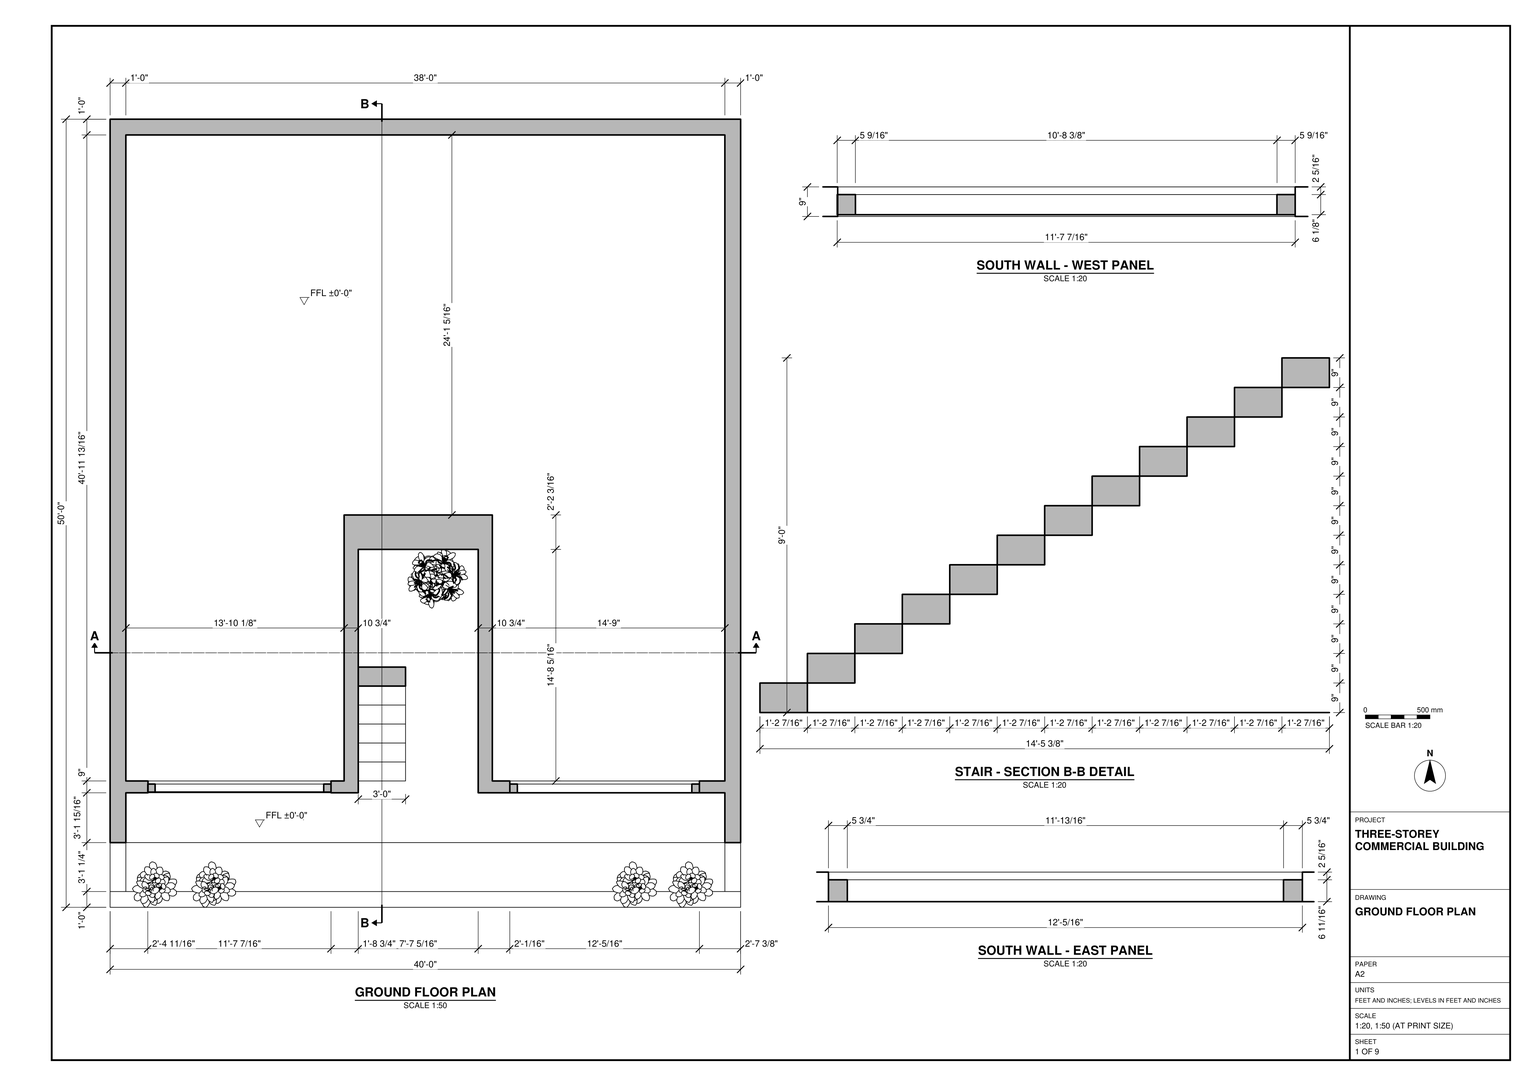
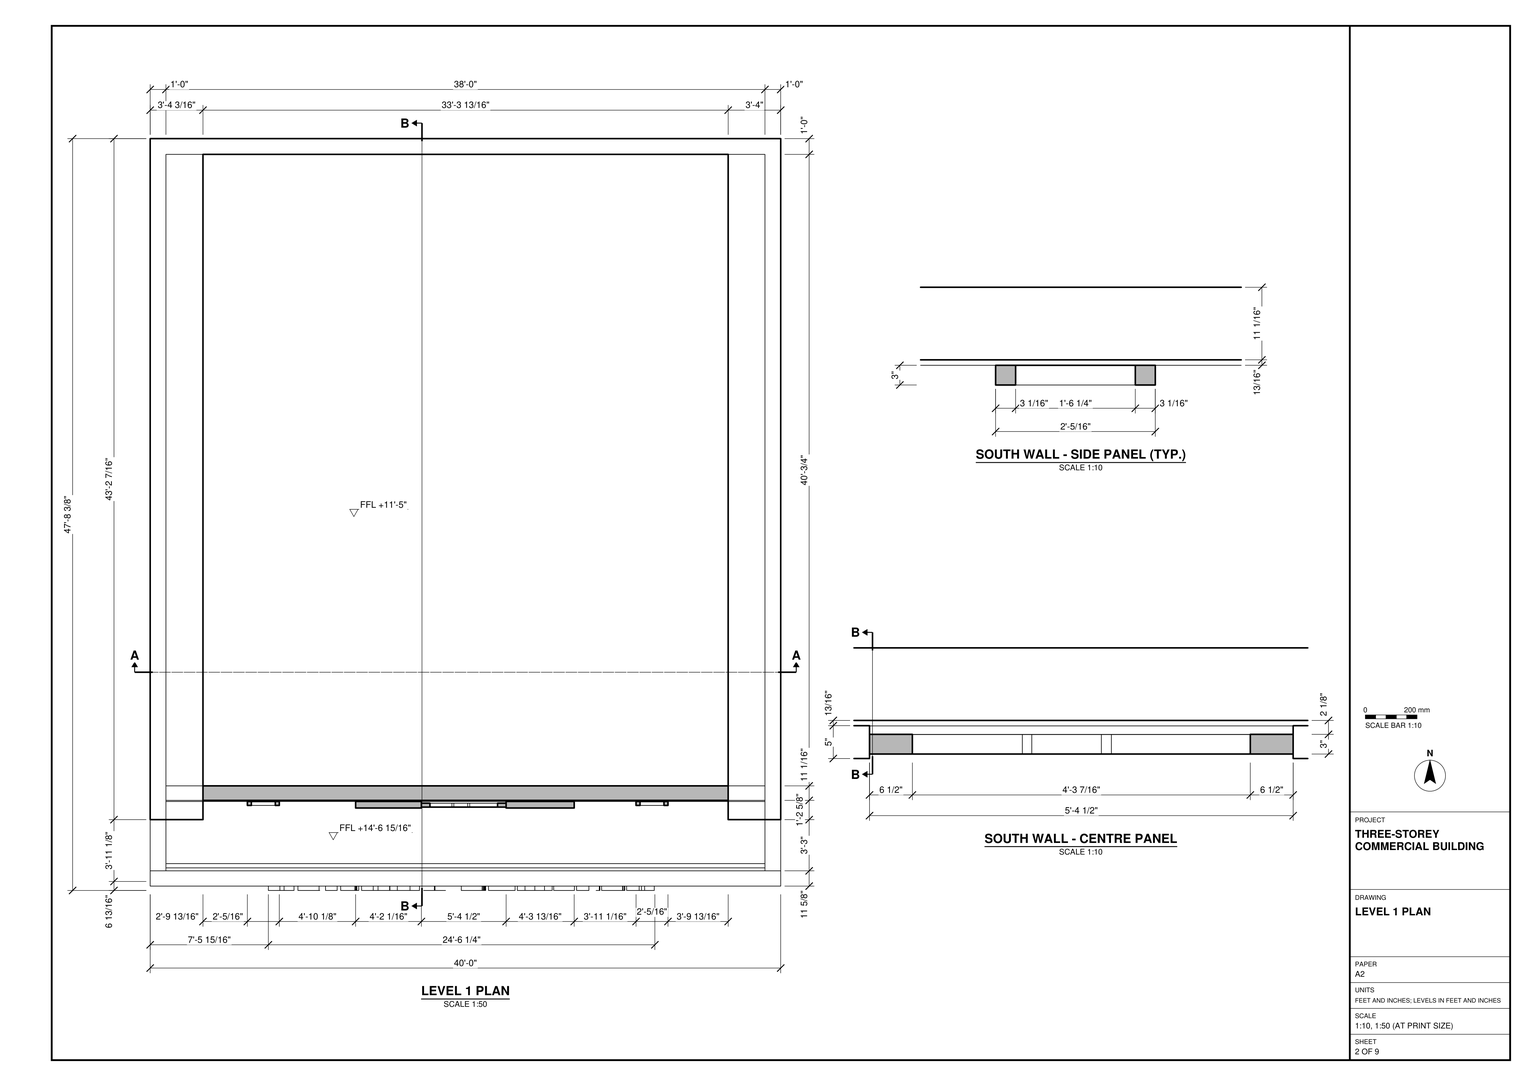
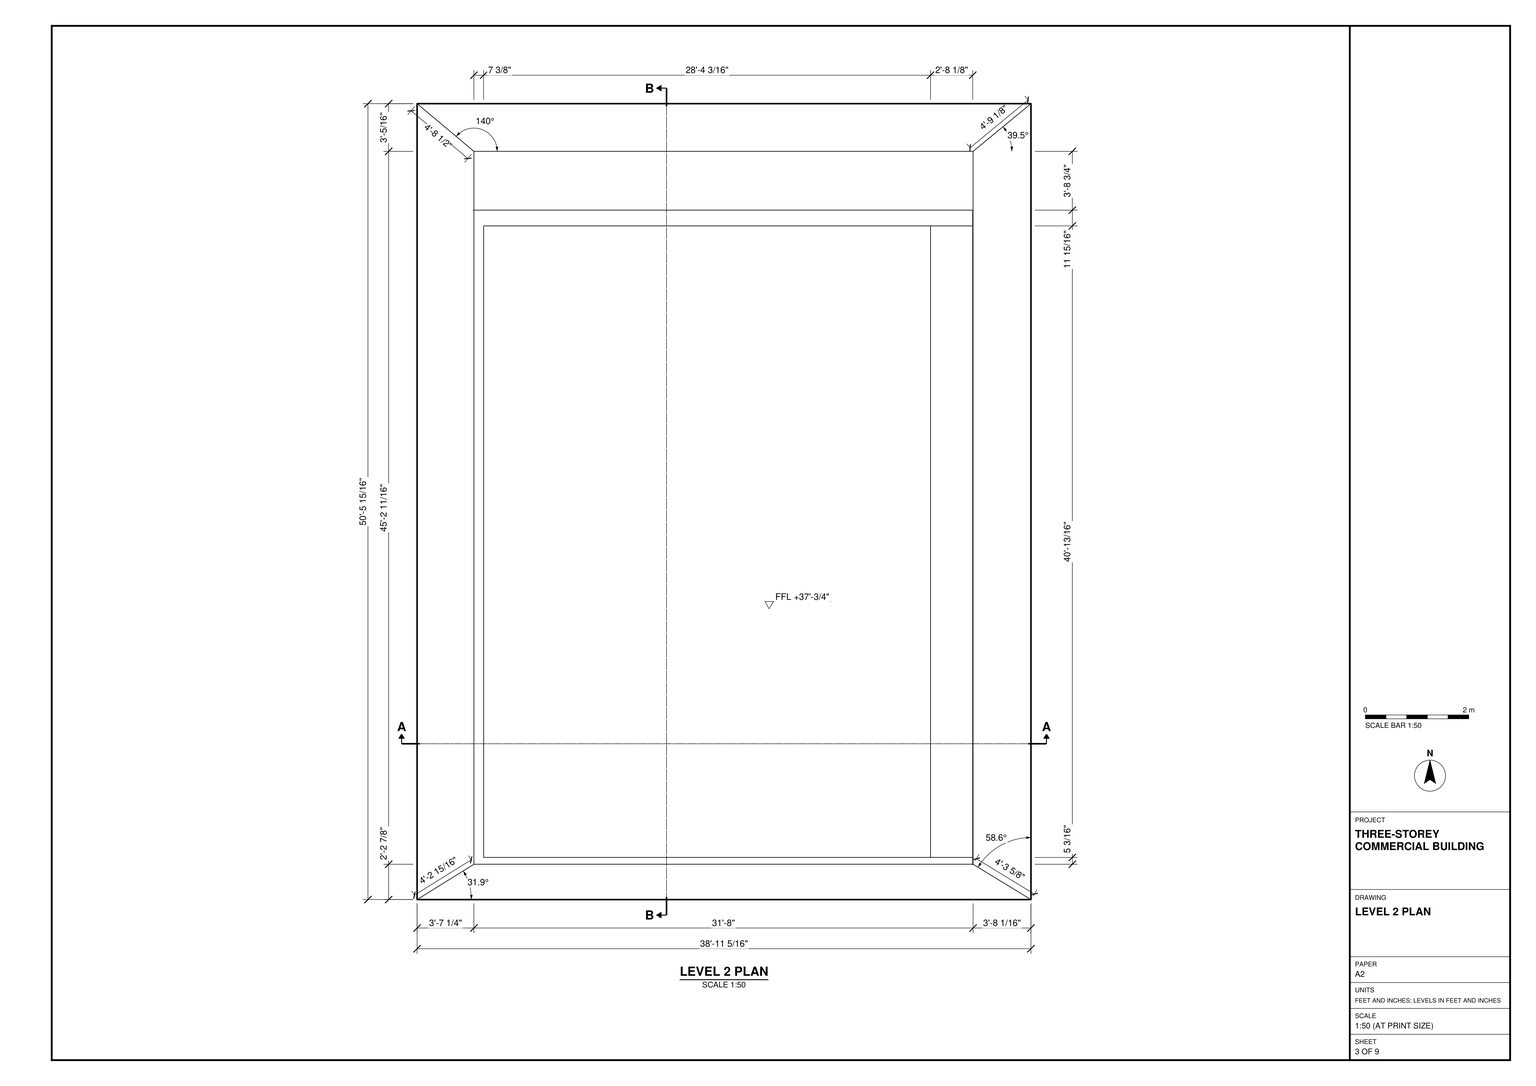
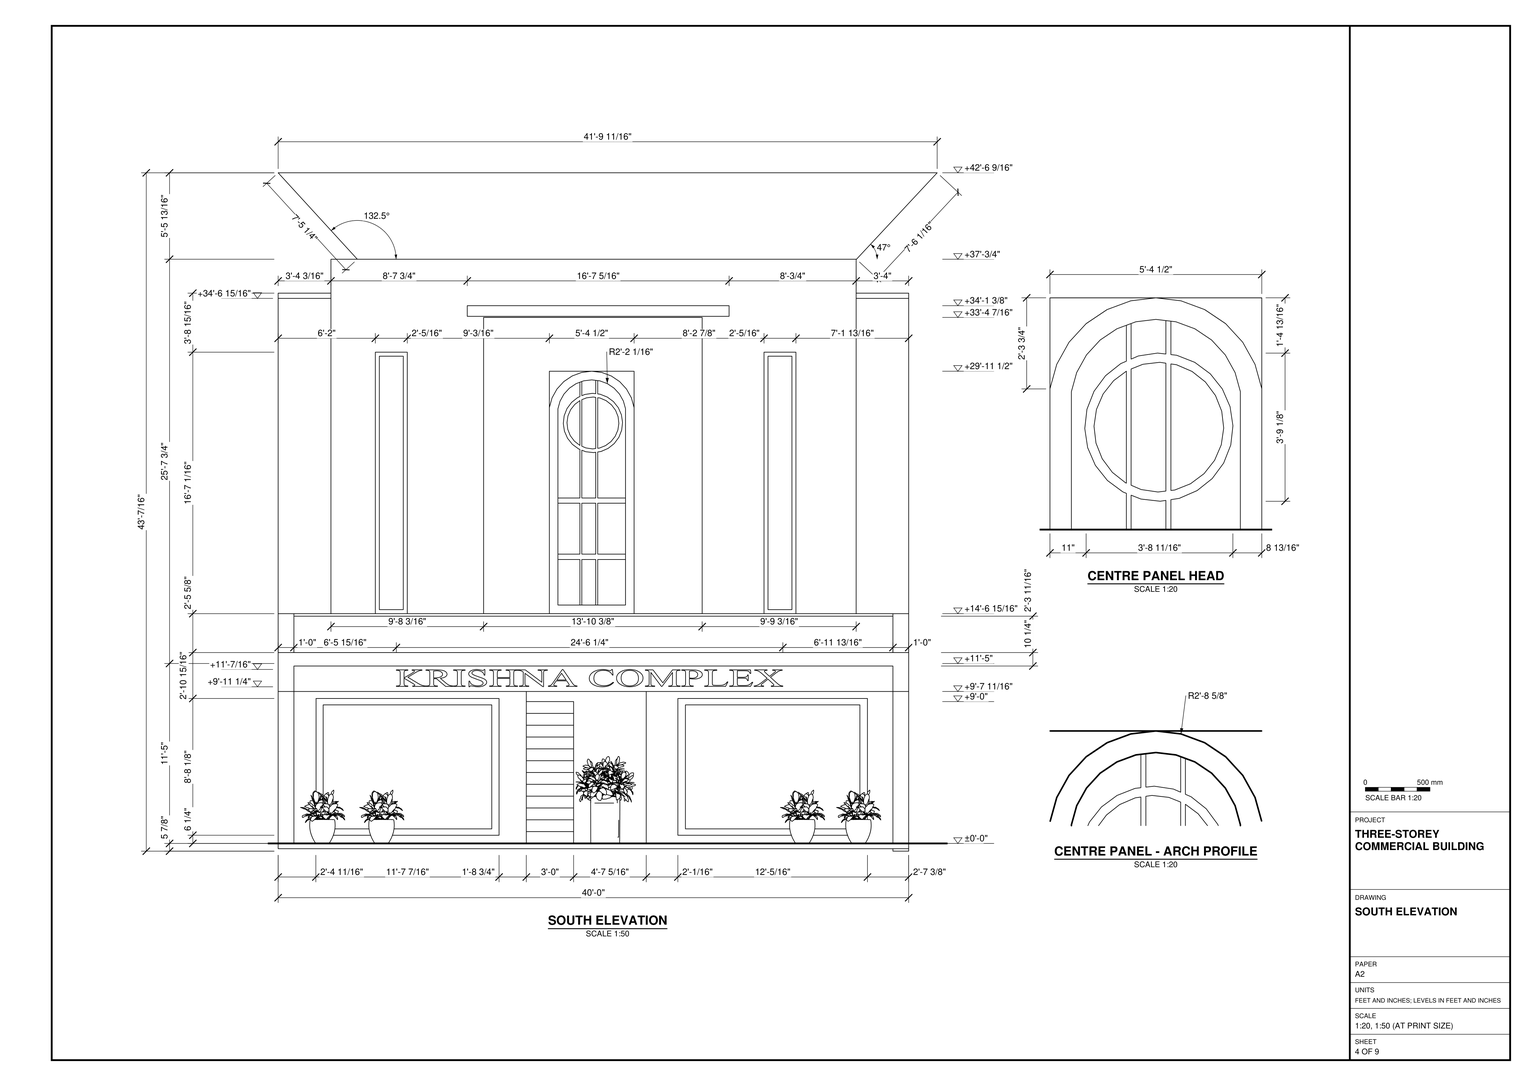
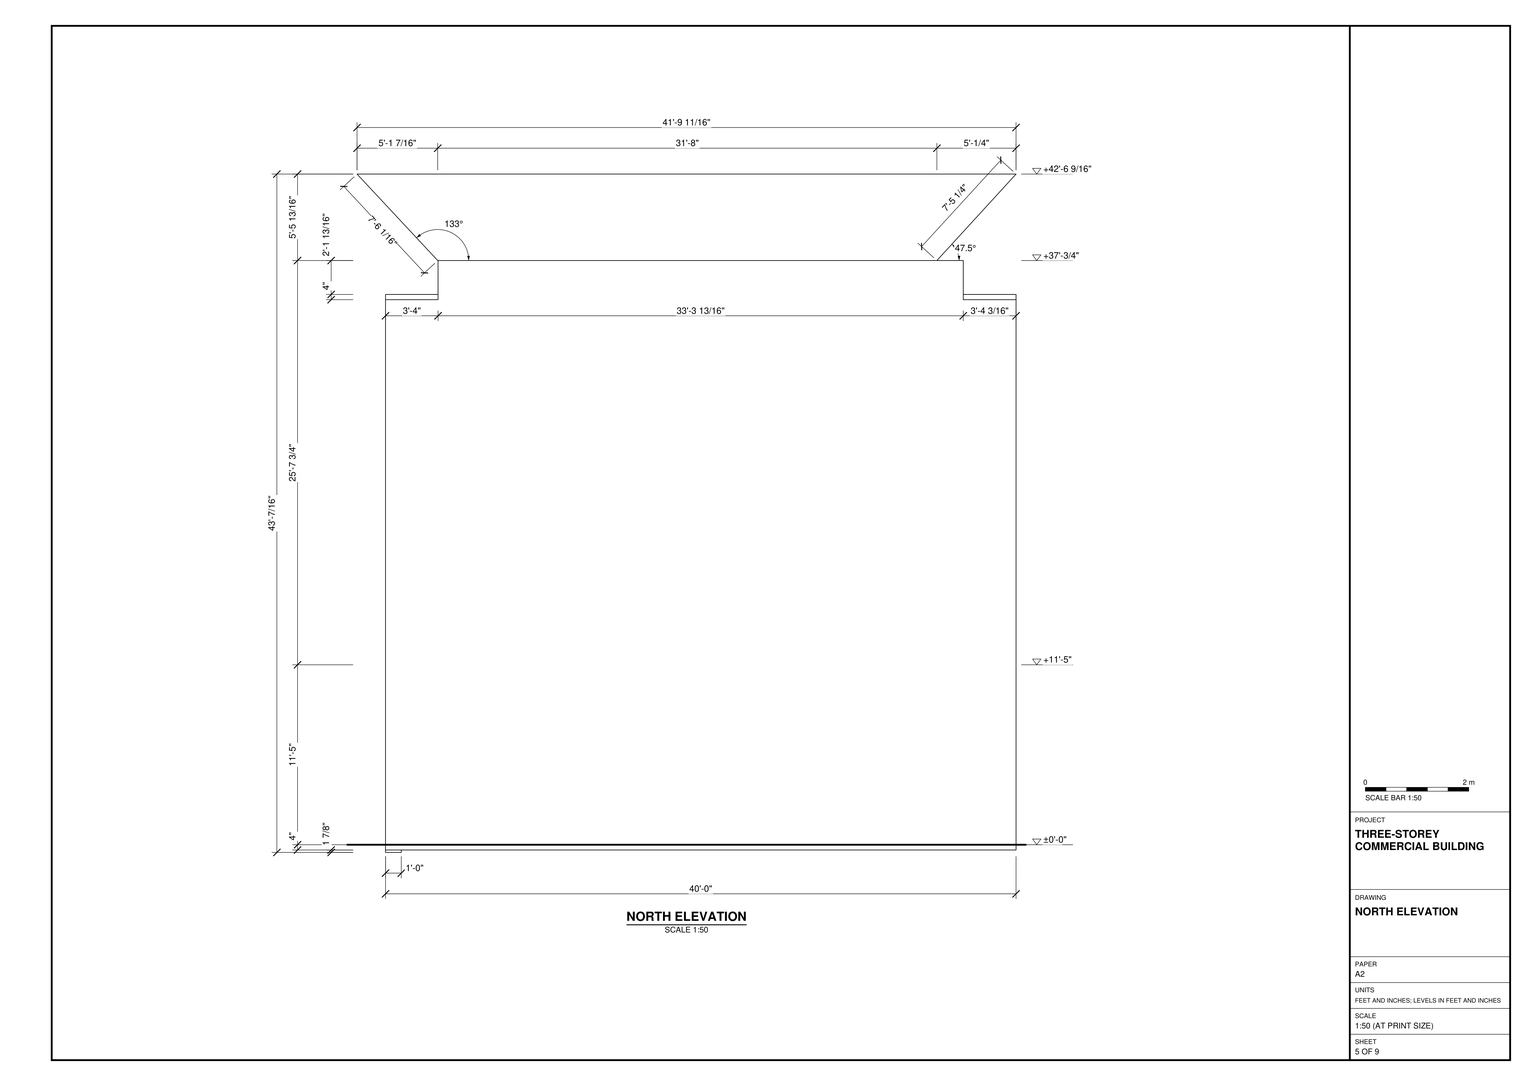
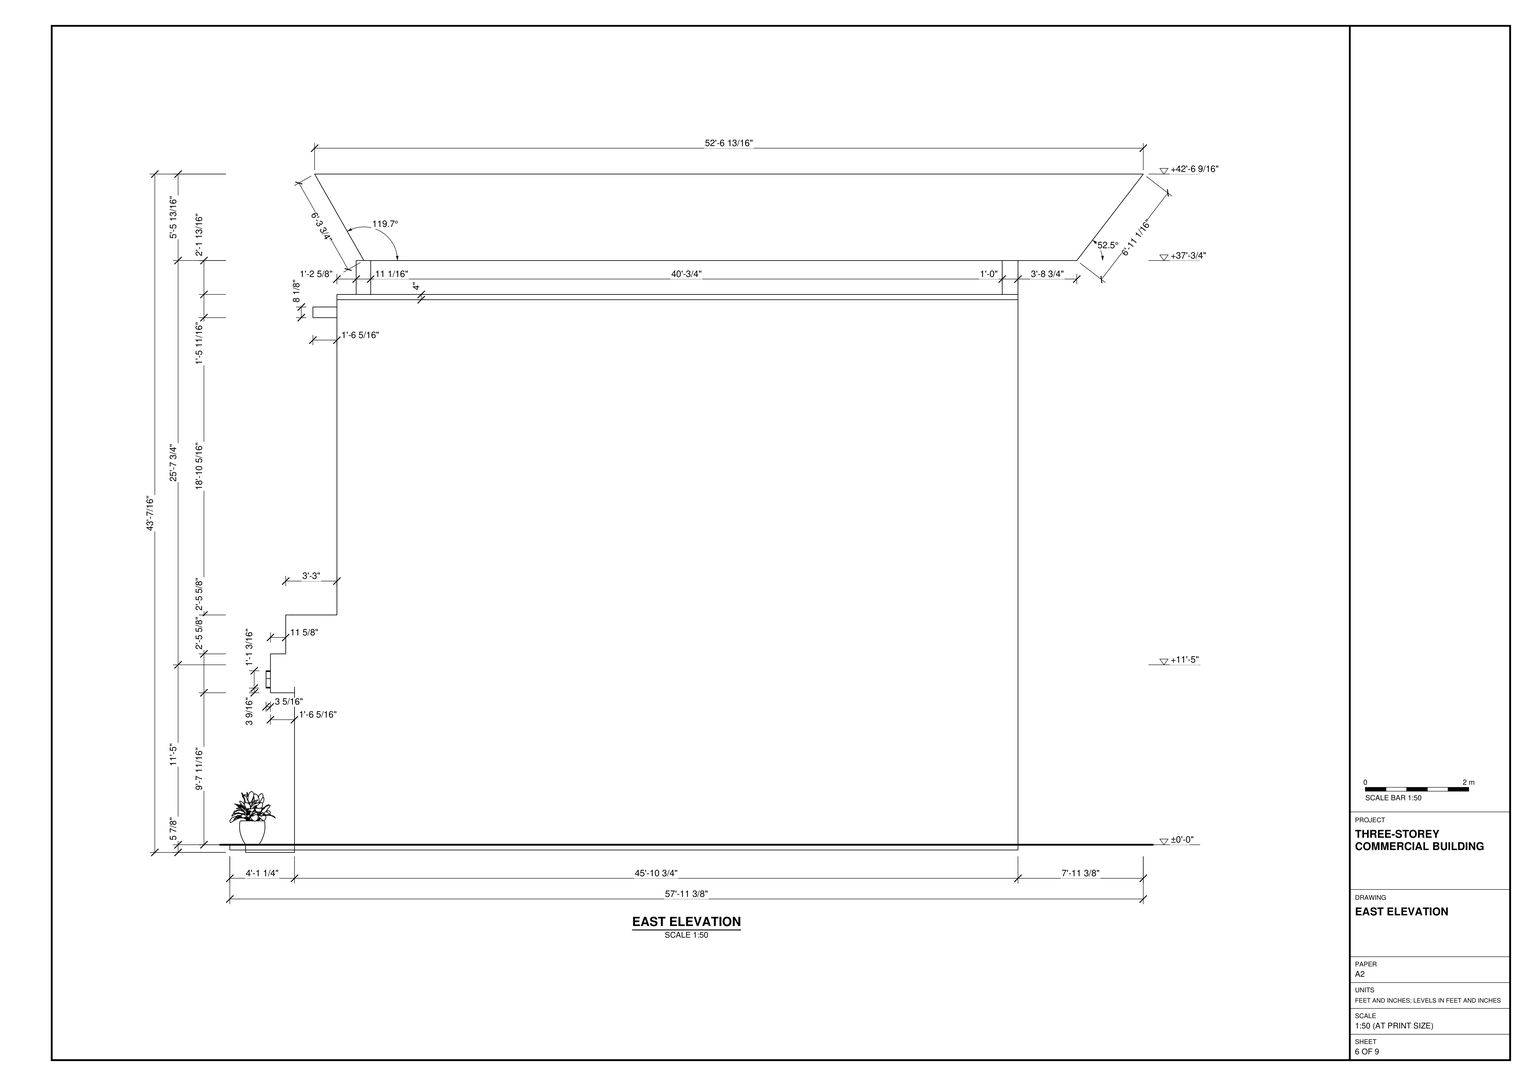
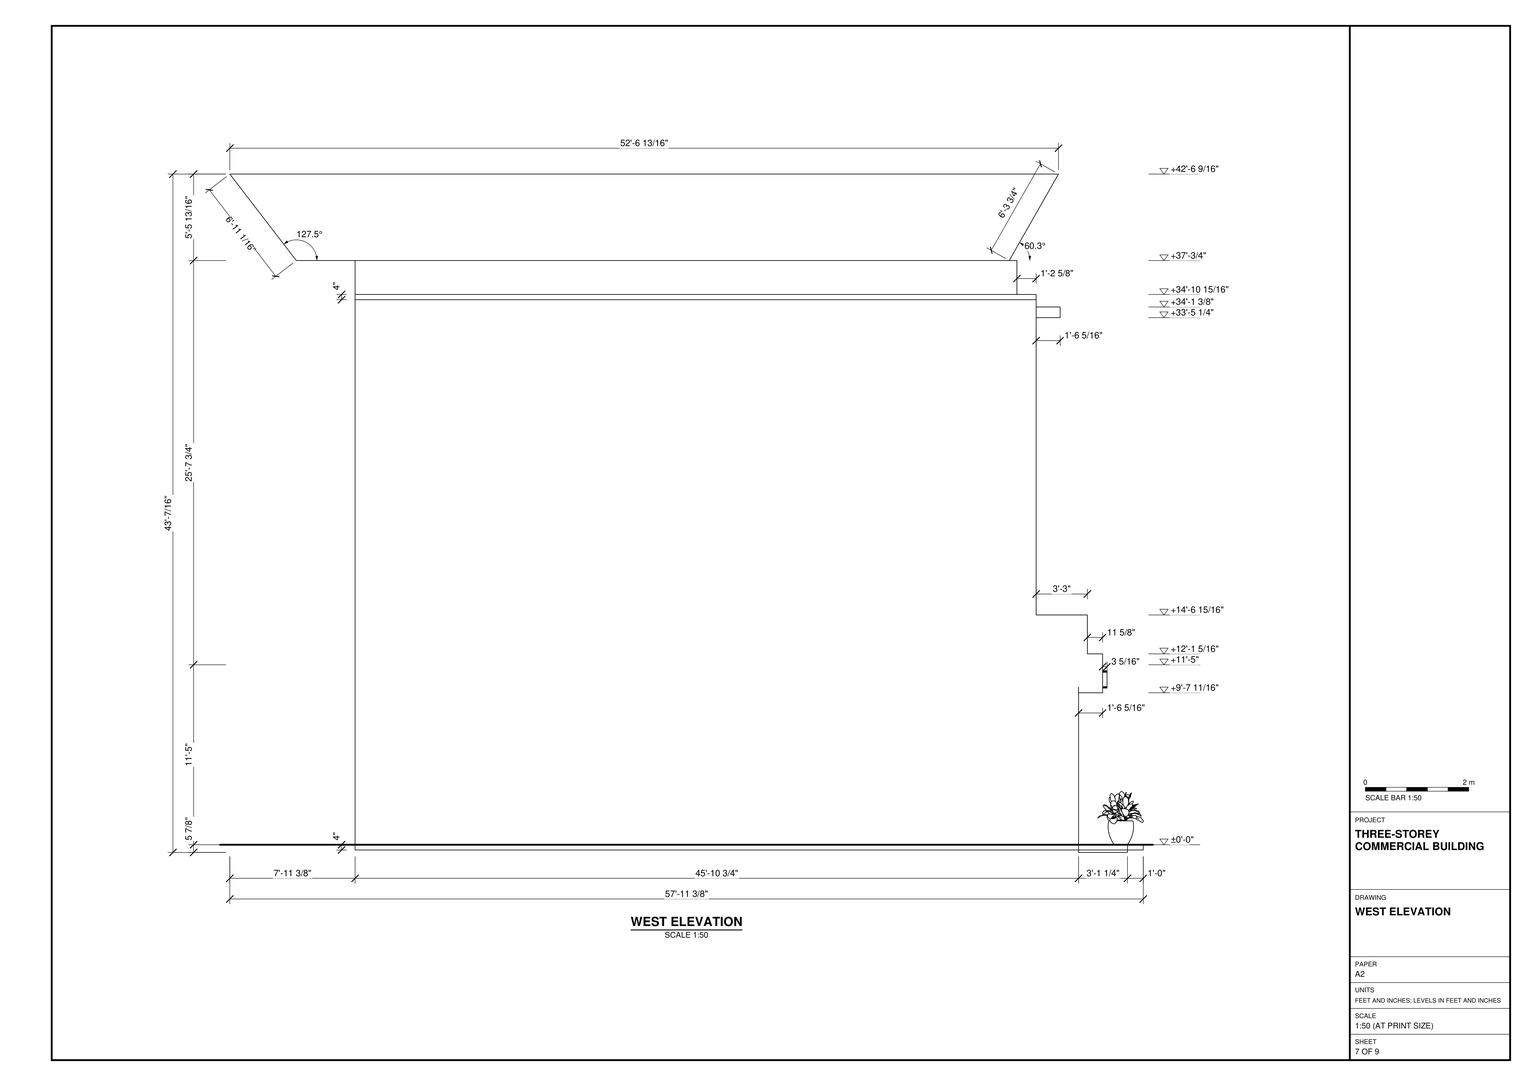
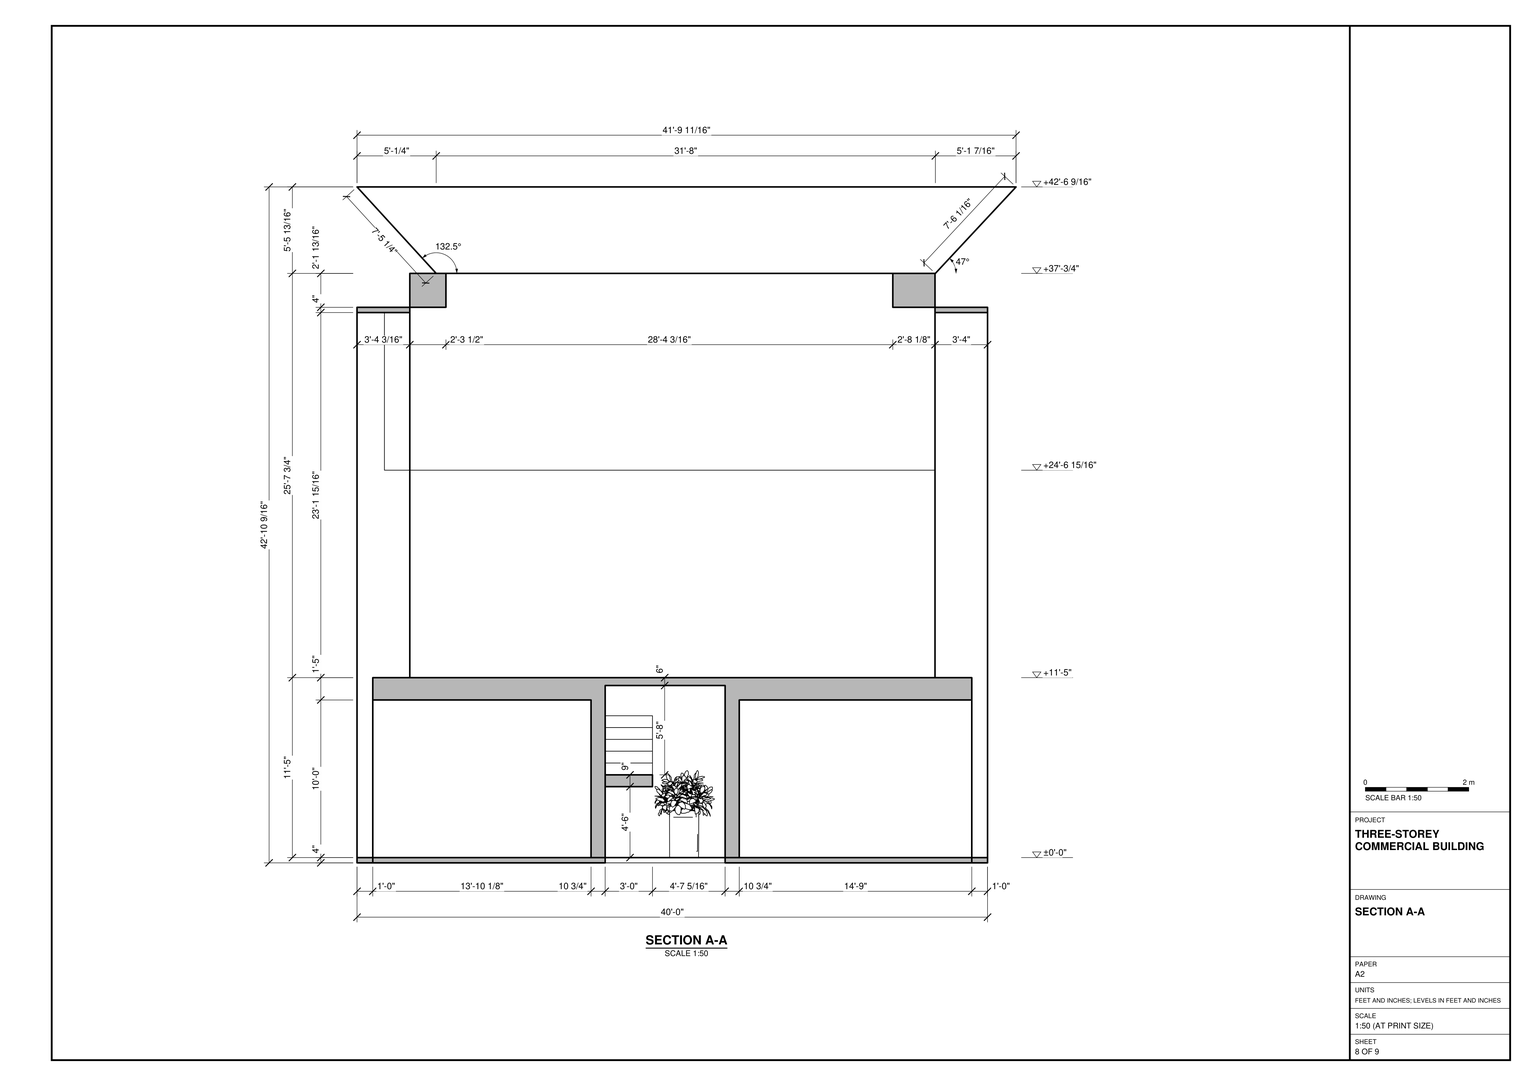
Build the three-storey commercial building in SketchUp using task_files/diagram_01.pdf. Work in feet and inches. The finished model must measure 41'-9 11/16" across X, 57'-11 3/8" along Y and 43'-7/16" high. Use ±0'-0" for the ground floor, +11'-5" for Level 1 and +37'-3/4" for Level 2.

Lay out the rectangular ground floor with the entrance facing south. Keep the broad interior open and form the entrance recess with wall returns on both sides. Place the straight stair along the west side of the recess and the framed wall panels on either side of its mouth. Follow the drawn wall thicknesses, panel widths and stair section. Include the front strip and place the planting where shown on the ground-floor plan.

Model the floor slabs, upper walls, openings and roof from the plans and sections. Set out the centre and side panels along the Level 1 south wall. At Level 2, distinguish the inset rectangular area from the perimeter band and follow the corner junctions in plan. Decor and loose items, including plants, may be any suitable library components.

Keep walls, slabs, roof and each furniture or joinery piece shown as separate groups or components, and use components for repeated parts. Save one SketchUp model as output_files/three_storey_commercial_building_with_recessed_entrance.skp.

# SketchUp Ruby script. Lengths in inches.
U = 1.inch
M = Sketchup.active_model
def pt(a) = Geom::Point3d.new(a.map { |v| v * U })
def face(e, loops, mat)
  f = e.add_face(loops[0].map { |a| pt(a) })
  loops[1..].each { |l| e.add_face(l.map { |a| pt(a) }).erase! }
  f.material = f.back_material = mat if mat
  f
end
# faces: each face lists its corners as indices into pts; further lists are holes
def faces(e, pts, list, mat = nil) = list.each { |f| face(e, (f[0].is_a?(Array) ? f : [f]).map { |l| l.map { |i| pts[i] } }, mat) }
# xy, xz, yz: faces in a plane at the given z, y or x. An outline is a flat list of corners, or four numbers for a rectangle; further outlines are holes
def ring(l) = l.size == 4 ? [[l[0], l[1]], [l[2], l[1]], [l[2], l[3]], [l[0], l[3]]] : l.each_slice(2).to_a
def flat(e, list, mat, &to3) = list.each { |f| face(e, (f[0].is_a?(Array) ? f : [f]).map { |l| ring(l).map { |u, v| to3.(u, v) } }, mat) }
def xy(e, z, list, mat = nil) = flat(e, list, mat) { |x, y| [x, y, z] }
def xz(e, y, list, mat = nil) = flat(e, list, mat) { |x, z| [x, y, z] }
def yz(e, x, list, mat = nil) = flat(e, list, mat) { |y, z| [x, y, z] }
def lines(e, pts, list) = list.each { |a, b| e.add_line(pt(pts[a]), pt(pts[b])) }
# prism: a flat outline (further loops are holes) pulled along v
def prism(e, loops, v, mat = nil)
  f = face(e, loops, mat); d = Geom::Vector3d.new(v.map { |x| x * U })
  f.pushpull(f.normal.samedirection?(d) ? d.length : -d.length)
end
def box(e, o, s, mat = nil) = prism(e, [[o, [o[0] + s[0], o[1], o[2]], [o[0] + s[0], o[1] + s[1], o[2]], [o[0], o[1] + s[1], o[2]]]], [0, 0, s[2]], mat)
def at(x, y, z, deg = 0) = Geom::Transformation.translation(pt([x, y, z])) * Geom::Transformation.rotation(ORIGIN, Z_AXIS, deg.degrees)
def axes(o, x, y, z) = Geom::Transformation.new([*x, 0, *y, 0, *z, 0, *pt(o).to_a, 1])
def part(name) = M.definitions.add(name)
# library, detail: a bought-in or finely detailed component or shape, given as its bounding box
def library(name, o, s) = part(name).tap { |d| box(d.entities, o, s) }
def detail(e, o, s) = box(e.add_group.entities, o, s)
def put(e, d, t, mat = nil) = e.add_instance(d, t).tap { |i| i.material = mat if mat }
def group(e, t, mat = nil) = e.add_group.tap { |g| g.transformation = t; g.material = mat if mat }.entities
root = M.entities
M.materials.add("[Brick Tumbled]").color = [135, 132, 132]
M.materials.add("[Color C08]").color = [102, 51, 0]
M.materials.add("[Color E06]").color = [204, 204, 0]
M.materials.add("[Color M01]").color = [226, 226, 226]
M.materials.add("[Color M02]").color = [198, 198, 198]
M.materials.add("[Color M05]").color = [114, 114, 114]
M.materials.add("[Grass Dark Green]").color = [106, 157, 55]
M.materials.add("[Stone Vein Gray]").color = [166, 165, 165]
M.materials.add("[Translucent Glass Dark Green]").color = [62, 91, 5]
M.materials["[Translucent Glass Dark Green]"].alpha = 0.5
M.materials.add("[Translucent Glass Gray]").color = [128, 128, 128]
M.materials["[Translucent Glass Gray]"].alpha = 0.5
M.materials.add("[Wood Fence]").color = [142, 67, 30]
c1 = library("PLANTS 75",[-21.16,-23.68,0],[45.42,44.51,66.32])
c2 = library("KRISHNA COMPLEX",[0.57,0,0],[326.93,23.97,4])
c3 = library("PLANTS 75\#1",[-17.06,-18.11,0],[33.69,34.67,40.66])
c4 = part("Group\#1")
box(c4.entities,[0,0,0],[36,17,6])
c5 = part("Group\#5")
xy(c5.entities,0,[[0,0,24.3125,3]],"[Color C08]")
xy(c5.entities,3.04,[[3.04,0,21.27,3]],"[Color C08]")
xy(c5.entities,196.02,[[3.04,0,21.27,3]],"[Color C08]")
xy(c5.entities,199.0625,[[0,0,24.3125,3]],"[Color C08]")
xz(c5.entities,0,[[[0,0,24.3125,199.0625],[3.04,3.04,21.27,196.02]]],"[Color C08]")
xz(c5.entities,3,[[[0,0,24.3125,199.0625],[3.04,3.04,21.27,196.02]]],"[Color C08]")
xz(c5.entities,3,[[3.04,3.04,21.27,196.02]],"[Translucent Glass Dark Green]")
yz(c5.entities,0,[[0,0,3,199.0625]],"[Color C08]")
yz(c5.entities,3.04,[[0,3.04,3,196.02]],"[Color C08]")
yz(c5.entities,21.27,[[0,3.04,3,196.02]],"[Color C08]")
yz(c5.entities,24.3125,[[0,0,3,199.0625]],"[Color C08]")
c6 = part("Group\#6")
xy(c6.entities,0,[[0,0,145.3125,9]],"[Color C08]")
xy(c6.entities,5.79,[[5.79,0,139.52,9]],"[Color C08]")
xy(c6.entities,118.21,[[5.79,0,139.52,9]],"[Color C08]")
xy(c6.entities,124,[[0,0,145.3125,9]],"[Color C08]")
xz(c6.entities,0,[[[0,0,145.3125,124],[5.79,5.79,139.52,118.21]]],"[Color C08]")
xz(c6.entities,0,[[5.79,5.79,139.52,118.21]],"[Translucent Glass Gray]")
xz(c6.entities,9,[[[0,0,145.3125,124],[5.79,5.79,139.52,118.21]]],"[Color C08]")
yz(c6.entities,0,[[0,0,9,124]],"[Color C08]")
yz(c6.entities,5.79,[[0,5.79,9,118.21]],"[Color C08]")
yz(c6.entities,139.52,[[0,5.79,9,118.21]],"[Color C08]")
yz(c6.entities,145.3125,[[0,0,9,124]],"[Color C08]")
xy(root,-1.875,[[468,12,480,49.25]])
xy(root,0,[[0,0,480,12],[0,12,12,49.25],[468,12,468,87.1875,280.21,87.1875,280.21,96.1875,468,96.1875,468,588,12,588,12,96.1875,188.91,96.1875,188.91,87.1875,12,87.1875,12,49.25,0,49.25,0,600,480,600,480,12],[12,12,468,87.1875],[188.91,87.1875,280.21,96.1875],
  [12,96.1875,12,588,468,588,468,96.1875,280.21,96.1875,280.21,272.48,188.91,272.48,188.91,96.1875]])
xy(root,4,[[0,49.25,0,600,480,600,480,49.25,468,49.25,468,87.1875,280.21,87.1875,280.21,96.1875,468,96.1875,468,588,12,588,12,96.1875,188.91,96.1875,188.91,87.1875,12,87.1875,12,49.25],[12,96.1875,178.15,96.1875,178.15,298.6875,290.98,298.6875,290.98,96.1875,468,96.1875,468,588,12,588],[178.15,96.1875,188.91,96.1875,188.91,272.48,280.21,272.48,280.21,96.1875,290.98,96.1875,290.98,298.6875,178.15,298.6875]])
xy(root,4,[[12,12,468,49.25]],"[Grass Dark Green]")
xy(root,4,[[0,0,480,12],[0,12,12,49.25],[468,12,480,49.25],[12,49.25,468,49.25,468,87.1875,280.21,87.1875,280.21,272.48,188.91,272.48,188.91,87.1875,12,87.1875]],"[Stone Vein Gray]")
xy(root,10.23,[[28.86,87.1875,168.17,96.1875],[304.29,87.1875,448.61,96.1875]])
xy(root,114.35,[[28.86,87.1875,168.17,96.1875],[304.29,87.1875,448.61,96.1875]])
xy(root,119.6875,[[0,30.9375,12,49.25],[468,30.9375,480,49.25],[12,34.4375,188.91,87.1875],[188.91,34.4375,280.21,87.1875],[280.21,34.4375,468,87.1875]])
xy(root,124,[[12,96.1875,12,588,468,588,468,96.1875,290.98,96.1875,290.98,298.6875,178.15,298.6875,178.15,96.1875]])
xy(root,135,[[188.91,87.1875,280.21,272.48]])
xy(root,139.07,[[12,30.9375,468,34.4375]])
xy(root,141,[[12,42.5625,468,72.9375],[12,72.9375,188.91,87.1875],[188.91,72.9375,280.21,87.1875],[280.21,72.9375,468,87.1875],[12,87.1875,468,96.1875],
  [12,96.1875,40.1875,107.24],[440,96.1875,468,107.24],[12,107.24,40.1875,588],[40.1875,107.24,440,588],[440,107.24,468,588]])
xy(root,149.3125,[[0,30.9375,480,42.5625]])
xy(root,177,[[12,44.8125,468,72.9375],[12,72.9375,468,96.1875]])
xy(root,178.9375,[[12,48.05,468,48.05,468,81.54,440,81.54,440,95.36,40.1875,95.36,40.1875,81.54,12,81.54],[12,81.54,40.1875,95.36],[440,81.54,468,95.36]])
xy(root,178.9375,[[0,42.5625,12,81.54],[468,42.5625,480,81.54]],"[Color M05]")
xy(root,405.28,[[143.97,63.25,343.28,96.1875]],"[Color M02]")
xy(root,413.4,[[143.97,63.25,343.28,96.1875]],"[Color M02]")
xy(root,418.9375,[[0,81.54,40.1875,600],[440,81.54,480,600]])
xy(root,422.9375,[[0,81.54,40.1875,600],[440,81.54,480,600],[40.1875,107.24,67.6875,561.27],[407.875,107.24,440,588],[40.1875,561.27,67.6875,574.96],
  [40.1875,574.96,67.6875,588]])
xy(root,448.75,[[40.1875,96.1875,440,96.1875,440,107.24,67.6875,107.24,67.6875,588,440,588,440,600,40.1875,600],[67.6875,107.24,407.875,588],[407.875,107.24,440,588]])
xz(root,0,[[0,0,480,4]])
xz(root,12,[[468,-1.875,480,0],[0,0,12,4],[12,0,468,4],[468,0,480,4]])
xz(root,30.9375,[[0,119.6875,12,119.6875,12,139.07,468,139.07,468,119.6875,480,119.6875,480,149.3125,0,149.3125]],"[Color M05]")
xz(root,34.4375,[[12,119.6875,468,139.07]])
xz(root,42.5625,[[12,141,188.91,149.3125],[188.91,141,280.21,149.3125],[280.21,141,468,149.3125]])
xz(root,42.5625,[[0,149.3125,12,178.9375],[468,149.3125,480,178.9375]],"[Color M05]")
xz(root,49.25,[[468,-1.875,480,4],[0,0,12,4],[0,119.6875,12,124],[468,119.6875,480,124]])
xz(root,49.25,[[0,4,12,119.6875],[468,4,480,119.6875]],"[Color M05]")
xz(root,63.25,[[143.97,405.28,343.28,413.4]],"[Color M02]")
xz(root,72.9375,[[12,141,468,177]],"[Wood Fence]")
xz(root,81.54,[[0,418.9375,40.1875,422.9375],[440,418.9375,480,422.9375]])
xz(root,81.54,[[0,178.9375,40.1875,418.9375],[440,178.9375,480,418.9375]],"[Color M05]")
xz(root,87.1875,[[12,0,188.91,4],[280.21,0,468,4],[12,119.6875,188.91,124],[188.91,119.6875,280.21,135],[280.21,119.6875,468,124],
  [12,124,188.91,141],[280.21,124,468,141],[188.91,135,280.21,141]])
xz(root,87.1875,[[[12,4,188.91,119.6875],[28.86,10.23,168.17,114.35]],[[280.21,4,468,119.6875],[304.29,10.23,448.61,114.35]]],"[Color M05]")
xz(root,96.1875,[[12,0,188.91,4],[[12,4,178.15,124],[28.86,10.23,168.17,114.35]],[[290.98,4,468,124],[304.29,10.23,448.61,114.35]],[12,124,178.15,141],[290.98,124,468,141],
  [12,141,40.1875,177],[40.1875,141,178.15,177],[178.15,141,290.98,177],[290.98,141,440,177],[440,141,468,177],
  [143.97,405.28,343.28,413.4]])
xz(root,96.1875,[[[40.1875,177,440,448.75],[143.97,405.28,343.28,413.4]]],"[Color M02]")
xz(root,107.24,[[40.1875,141,40.1875,422.9375,67.6875,422.9375,67.6875,448.75,407.875,448.75,407.875,422.9375,440,422.9375,440,141],[407.875,422.9375,440,448.75]])
xz(root,272.48,[[188.91,0,280.21,4]])
xz(root,272.48,[[188.91,4,280.21,135]],"[Color M05]")
xz(root,298.6875,[[178.15,4,290.98,124]])
xz(root,588,[[12,0,468,4],[12,4,468,124],[12,124,20.875,141],[20.875,124,468,141],[40.1875,141,440,298.9375],
  [40.1875,298.9375,440,298.9375,440,422.9375,407.875,422.9375,407.875,448.75,67.6875,448.75,67.6875,422.9375,40.1875,422.9375],[407.875,422.9375,440,448.75]])
xz(root,600,[[0,0,480,4],[0,418.9375,40.1875,422.9375],[440,418.9375,480,422.9375]])
xz(root,600,[[0,4,0,418.9375,40.1875,418.9375,40.1875,448.75,440,448.75,440,418.9375,480,418.9375,480,4]],"[Color M05]")
yz(root,0,[[0,0,12,4],[12,0,49.25,4],[49.25,0,600,4],[81.54,418.9375,600,422.9375]])
yz(root,0,[[49.25,4,49.25,119.6875,30.9375,119.6875,30.9375,149.3125,42.5625,149.3125,42.5625,178.9375,81.54,178.9375,81.54,418.9375,600,418.9375,600,4]],"[Color M05]")
yz(root,12,[[12,0,49.25,4],[49.25,0,87.1875,4],[96.1875,0,588,4],[96.1875,4,588,124],[30.9375,119.6875,34.4375,139.07],
  [49.25,119.6875,87.1875,124],[96.1875,124,588,141],[72.9375,141,87.1875,177],[87.1875,141,96.1875,177],[44.8125,177,87.1875,177,87.07,178.9375,48.05,178.9375],
  [87.1875,177,96.1875,177,95.36,178.9375,87.07,178.9375]])
yz(root,12,[[49.25,4,87.1875,119.6875],[42.5625,141,72.9375,141,72.9375,177,44.8125,177,48.05,178.9375,42.5625,178.9375]],"[Color M05]")
yz(root,28.86,[[87.1875,10.23,96.1875,114.35]])
yz(root,40.1875,[[96.1875,141,107.24,298.9375],[107.24,141,588,298.9375],[96.1875,298.9375,107.24,418.9375],[107.24,298.9375,588,418.9375],[81.54,418.9375,96.1875,422.9375],
  [96.1875,418.9375,107.24,422.9375],[107.24,418.9375,588,422.9375],[588,418.9375,600,422.9375],[96.1875,422.9375,600,448.75]])
yz(root,40.1875,[[96.1875,177,96.1875,418.9375,81.54,418.9375,81.54,178.9375,95.36,178.9375]],"[Color M05]")
yz(root,67.6875,[[107.24,422.9375,588,448.75]])
yz(root,143.97,[[63.25,405.28,96.1875,413.4]],"[Color M01]")
yz(root,156.4,[[95.36,178.9375,90.36,178.96,91.1875,404.47,96.1875,404.45]],"[Color M02]")
yz(root,168.17,[[87.1875,10.23,96.1875,114.35]])
yz(root,178.15,[[96.1875,4,298.6875,124]])
yz(root,188.91,[[87.1875,0,96.1875,4],[96.1875,0,272.48,4]])
yz(root,188.91,[[87.1875,4,272.48,135]],"[Color M05]")
yz(root,206.46,[[95.36,178.9375,96.04,363.48,91.04,363.5,90.36,178.96]])
yz(root,270.96,[[95.36,178.9375,90.36,178.96,91.04,363.5,96.04,363.48]])
yz(root,280.21,[[87.1875,0,96.1875,4],[96.1875,0,272.48,4],[87.1875,4,272.48,135]])
yz(root,290.98,[[96.1875,4,298.6875,124]])
yz(root,304.29,[[87.1875,10.23,96.1875,114.35]])
yz(root,322.79,[[95.36,178.9375,96.1875,404.45,91.1875,404.47,90.36,178.96]],"[Color M02]")
yz(root,343.28,[[63.25,405.28,96.1875,413.4]],"[Color M02]")
yz(root,407.875,[[107.24,422.9375,588,448.75]])
yz(root,440,[[96.1875,141,107.24,298.9375],[107.24,141,588,298.9375],[96.1875,298.9375,107.24,418.9375],[107.24,298.9375,588,418.9375],[81.54,418.9375,96.1875,422.9375],
  [96.1875,418.9375,107.24,422.9375],[107.24,418.9375,588,422.9375],[588,418.9375,600,422.9375],[96.1875,422.9375,107.24,448.75],[107.24,422.9375,588,448.75],
  [588,422.9375,600,448.75]])
yz(root,440,[[96.1875,177,95.36,178.9375,81.54,178.9375,81.54,418.9375,96.1875,418.9375]],"[Color M05]")
yz(root,448.61,[[87.1875,10.23,96.1875,114.35]])
yz(root,468,[[12,-1.875,49.25,0],[12,0,49.25,4],[49.25,0,87.1875,4],[96.1875,0,588,4],[96.1875,4,588,124],
  [30.9375,119.6875,34.4375,139.07],[49.25,119.6875,87.1875,124],[96.1875,124,588,141],[72.9375,141,87.1875,177],[87.1875,141,96.1875,177],
  [44.8125,177,48.05,178.9375,87.07,178.9375,87.1875,177],[87.1875,177,87.07,178.9375,95.36,178.9375,96.1875,177]])
yz(root,468,[[49.25,4,87.1875,119.6875],[42.5625,141,42.5625,178.9375,48.05,178.9375,44.8125,177,72.9375,177,72.9375,141]],"[Color M05]")
yz(root,480,[[12,-1.875,49.25,0],[0,0,12,4],[12,0,49.25,4],[49.25,0,600,4],[81.54,418.9375,600,422.9375]])
yz(root,480,[[49.25,4,600,4,600,418.9375,81.54,418.9375,81.54,178.9375,42.5625,178.9375,42.5625,149.3125,30.9375,149.3125,30.9375,119.6875,49.25,119.6875]],"[Color M05]")
p = [[12,44.8125,177],[468,44.8125,177],[468,48.05,178.9375],[12,48.05,178.9375],[12,96.1875,177],[12,95.36,178.9375],
  [40.1875,95.36,178.9375],[40.1875,96.1875,177],[322.79,95.36,178.9375],[440,95.36,178.9375],[440,96.1875,177],[290.98,96.1875,177],
  [178.15,96.1875,177],[156.4,95.36,178.9375],[206.46,95.36,178.9375],[270.96,95.36,178.9375],[468,95.36,178.9375],[468,96.1875,177],
  [206.46,90.36,178.96],[156.4,90.36,178.96],[270.96,90.36,178.96],[322.79,90.36,178.96],[156.4,96.1875,404.45],[322.79,96.1875,404.45],
  [270.96,96.04,363.48],[206.46,96.04,363.48],[206.46,91.04,363.5],[270.96,91.04,363.5],[322.79,91.1875,404.47],[156.4,91.1875,404.47],
  [290.98,298.6875,124],[290.98,298.6875,141],[178.15,298.6875,124],[178.15,298.6875,141],[280.21,272.48,135],[280.21,272.48,141],
  [188.91,272.48,135],[188.91,272.48,141],[219.07,272.48,135],[219.07,272.48,141],[20.875,588,298.9375],[20.875,588,418.9375],
  [40.1875,588,298.9375]]
faces(root,p,[[0,1,2,3],[4,5,6,7],[8,9,10,11,12,7,6,13,14,15],[16,17,10,9],[13,14,18,19],[20,15,8,21],[13,22,23,8,15,24,25,14],[27,26,25,24],
  [23,22,29,28]])
faces(root,p,[[19,18,26,27,20,21,28,29]],"[Brick Tumbled]")
lines(root,p,[[30,31],[32,33],[34,35],[36,37],[38,39],[40,41],[40,42]])
put(root,c1,at(247.87,251.38,4))
put(root,c2,axes([89.45,34.4375,123.26],[0.9,0,0],[0,0,0.55],[0,-1.71,0]),"[Color E06]")
put(root,c3,at(34.1,18.11,4))
put(root,c3,at(79.1,18.11,4))
put(root,c3,at(399.42,18.11,4))
put(root,c3,at(442.17,18.11,4))
g1 = group(root,at(188.91,96.18,4))
put(g1,c4,axes([0,28.9,18],[1,0,0],[0,0.85,0],[0,0,1.5]))
put(g1,c4,axes([0,101.15,63],[1,0,0],[0,0.85,0],[0,0,1.5]))
put(g1,c4,axes([0,130.05,81],[1,0,0],[0,0.85,0],[0,0,1.5]))
put(g1,c4,axes([0,57.8,36],[1,0,0],[0,0.85,0],[0,0,1.5]))
put(g1,c4,axes([0,158.95,99],[1,0,0],[0,0.85,0],[0,0,1.5]))
put(g1,c4,axes([0,115.6,72],[1,0,0],[0,0.85,0],[0,0,1.5]))
put(g1,c4,axes([0,43.35,27],[1,0,0],[0,0.85,0],[0,0,1.5]))
put(g1,c4,axes([0,72.25,45],[1,0,0],[0,0.85,0],[0,0,1.5]))
put(g1,c4,axes([0,86.7,54],[1,0,0],[0,0.85,0],[0,0,1.5]))
put(g1,c4,axes([0,0,0],[1,0,0],[0,0.85,0],[0,0,1.5]))
put(g1,c4,axes([0,144.5,90],[1,0,0],[0,0.85,0],[0,0,1.5]))
put(g1,c4,axes([0,14.45,9],[1,0,0],[0,0.85,0],[0,0,1.5]))
g2 = group(root,at(0,64.54,448.75),"[Color M01]")
xy(g2,0,[[60.28,37.49,440.25,580.22]])
xy(g2,65.83,[[0,0,501.69,630.82]])
p = [[0,630.82,65.83],[60.28,580.22,0],[60.28,37.49,0],[0,0,65.83],[440.25,37.49,0],[501.69,0,65.83],
  [440.25,580.22,0],[501.69,630.82,65.83]]
faces(g2,p,[[0,1,2,3],[4,5,3,2],[6,7,5,4],[0,7,6,1]])
g3 = group(root,at(206.46,91.04,178.94))
yz(g3,0,[[3,0,0,0.01,0.58,156.88,3.58,156.87]],"[Color C08]")
yz(g3,6.52,[[3.02,6.52,3.15,41.21,0.15,41.22,0.02,6.53],[3.15,41.21,3.17,45.29,0.17,45.3,0.15,41.22],[3.17,45.29,3.31,84.0625,0.31,84.07,0.17,45.3],[3.31,84.0625,3.32,88.01,0.32,88.02,0.31,84.07],[3.32,88.01,3.58,155.98,0.58,155.99,0.32,88.02]],"[Color C08]")
yz(g3,57.97,[[3.02,6.52,0.02,6.53,0.15,41.22,3.15,41.21],[3.15,41.21,0.15,41.22,0.17,45.3,3.17,45.29],[3.17,45.29,0.17,45.3,0.31,84.07,3.31,84.0625],[3.31,84.0625,0.31,84.07,0.32,88.02,3.32,88.01],[3.32,88.01,0.32,88.02,0.58,155.99,3.58,155.98]],"[Color C08]")
yz(g3,64.5,[[3,0,3.58,156.87,0.58,156.88,0,0.01]],"[Color C08]")
p = [[39.89,0.68,183.64],[32.25,0.68,184.55],[24.61,0.68,183.64],[17.39,0.67,180.97],[11,0.65,176.6875],[5.79,0.63,171.02],
  [2.06,0.61,164.3],[0,0.58,156.88],[0,0,0.01],[64.5,0,0.01],[64.5,0.58,156.88],[62.44,0.61,164.3],
  [58.7,0.63,171.02],[53.5,0.65,176.6875],[47.11,0.67,180.97],[15.28,0.63,171.7],[20.38,0.65,175.125],[23.27,0.65,176.19],
  [24.71,0.65,176.72],[26.15,0.65,177.26],[32.25,0.66,177.98],[35.3,0.66,177.62],[36.83,0.65,177.4375],[38.35,0.65,177.26],
  [44.11,0.65,175.125],[49.22,0.63,171.7],[53.375,0.62,167.18],[56.36,0.6,161.8],[57.97,0.58,155.99],[57.97,0.32,88.02],
  [57.97,0.31,84.07],[57.97,0.17,45.3],[57.97,0.15,41.22],[57.97,0.02,6.53],[36.83,0.02,6.53],[35.3,0.02,6.53],
  [24.71,0.02,6.53],[23.27,0.02,6.53],[6.52,0.02,6.53],[6.52,0.15,41.22],[6.52,0.17,45.3],[6.52,0.31,84.07],
  [6.52,0.32,88.02],[6.52,0.58,155.99],[8.14,0.6,161.8],[11.12,0.62,167.18],[0,3,0],[64.5,3,0],
  [32.25,3.68,184.54],[39.89,3.68,183.63],[47.11,3.67,180.96],[53.5,3.65,176.67],[58.7,3.63,171.01],[62.44,3.61,164.28],
  [64.5,3.58,156.87],[0,3.58,156.87],[2.06,3.61,164.28],[5.79,3.63,171.01],[11,3.65,176.67],[17.39,3.67,180.96],
  [24.61,3.68,183.63],[20.38,3.65,175.11],[15.28,3.63,171.6875],[11.12,3.62,167.17],[8.14,3.6,161.79],[6.52,3.58,155.98],
  [6.52,3.32,88.01],[6.52,3.31,84.0625],[6.52,3.17,45.29],[6.52,3.15,41.21],[6.52,3.02,6.52],[23.27,3.02,6.52],
  [24.71,3.02,6.52],[35.3,3.02,6.52],[36.83,3.02,6.52],[57.97,3.02,6.52],[57.97,3.15,41.21],[57.97,3.17,45.29],
  [57.97,3.31,84.0625],[57.97,3.32,88.01],[57.97,3.58,155.98],[56.36,3.6,161.79],[53.375,3.62,167.17],[49.22,3.63,171.6875],
  [44.11,3.65,175.11],[38.35,3.65,177.25],[36.83,3.65,177.43],[35.3,3.66,177.61],[32.25,3.66,177.97],[26.15,3.65,177.25],
  [24.71,3.65,176.71],[23.27,3.65,176.18],[23.27,0.15,41.22],[24.71,0.15,41.22],[35.3,0.15,41.22],[36.83,0.15,41.22],
  [36.83,0.17,45.3],[36.83,0.31,84.07],[36.83,0.32,88.02],[36.83,0.45,123.1],[39.38,0.46,123.48],[44.75,0.46,125.82],
  [44.78,0.46,125.83],[49.39,0.48,129.5],[52.89,0.5,134.24],[55.05,0.52,139.72],[55.71,0.54,145.57],[54.84,0.56,151.4],
  [52.49,0.58,156.8],[48.82,0.6,161.4],[44.08,0.61,164.91],[38.6,0.62,167.0625],[36.83,0.62,167.26],[35.3,0.62,167.4375],
  [32.75,0.62,167.73],[26.93,0.62,166.85],[24.71,0.61,165.89],[23.27,0.61,165.26],[21.53,0.61,164.5],[16.92,0.59,160.83],
  [13.42,0.58,156.1],[11.26,0.56,150.61],[10.6,0.53,144.76],[11.47,0.51,138.9375],[13.82,0.49,133.54],[17.49,0.48,128.93],
  [21.7,0.46,125.82],[22.23,0.46,125.43],[23.27,0.46,125.02],[23.27,0.32,88.02],[23.27,0.31,84.07],[23.27,0.17,45.3],
  [35.3,0.31,84.07],[35.3,0.17,45.3],[24.71,0.17,45.3],[24.71,0.31,84.07],[35.3,0.45,122.87],[35.3,0.32,88.02],
  [24.71,0.32,88.02],[24.71,0.46,124.45],[27.71,0.45,123.27],[33.56,0.45,122.61],[35.3,0.46,125.7],[35.3,0.61,164.64],
  [33.43,0.61,164.91],[28.3125,0.61,164.3125],[24.71,0.6,162.88],[24.71,0.47,127.49],[27.78,0.47,126.16],[30.16,0.46,125.82],
  [32.88,0.46,125.42],[36.83,0.61,164.42],[36.83,0.46,125.88],[38,0.47,126.02],[42.79,0.47,127.93],[46.92,0.48,131.01],
  [50.12,0.5,135.05],[52.16,0.52,139.79],[52.9,0.53,144.89],[52.3,0.55,150.01],[50.4,0.57,154.8],[47.32,0.59,158.93],
  [43.27,0.6,162.13],[38.53,0.61,164.17],[23.27,0.47,128.11],[23.27,0.6,162.22],[19.39,0.59,159.33],[16.19,0.57,155.28],
  [14.15,0.56,150.55],[13.41,0.54,145.44],[14.01,0.52,140.32],[15.91,0.5,135.53],[18.99,0.48,131.4],[23.04,0.47,128.2]]
faces(g3,p,[[[0,1,2,3,4,5,6,7,8,9,10,11,12,13,14],[15,16,17,18,19,20,21,22,23,24,25,26,27,28,29,30,31,32,33,34,35,36,37,38,39,40,41,42,43,44,45]],[[48,49,50,51,52,53,54,47,46,55,56,57,58,59,60],[61,62,63,64,65,66,67,68,69,70,71,72,73,74,75,76,77,78,79,80,81,82,83,84,85,86,87,88,89,90,91]],[[93,94,35,34,95,32,31,96,97,30,29,98,99,100,101,102,103,104,105,106,107,108,109,110,111,112,22,21,113,114,115,116,18,17,117,118,119,120,121,122,123,124,125,126,127,128,129,42,41,130,131,40,39,92,37,36],[132,133,134,135],[136,137,138,139,140,141]],[38,37,71,70],[37,36,72,71],[36,35,73,72],[35,34,74,73],[34,33,75,74],
  [44,43,65,64],[28,27,81,80],[7,6,56,55],[11,10,54,53],[45,44,64,63],[27,26,82,81],[6,5,57,56],[12,11,53,52],
  [15,45,63,62],[26,25,83,82],[5,4,58,57],[13,12,52,51],[16,15,62,61],[25,24,84,83],[17,16,61,91],[24,23,85,84],
  [18,17,91,90],[4,3,59,58],[19,18,90,89],[14,13,51,50],[20,19,89,88],[23,22,86,85],[22,21,87,86],[21,20,88,87],
  [3,2,60,59],[0,14,50,49],[2,1,48,60],[1,0,49,48]],"[Color C08]")
faces(g3,p,[[9,8,46,47]])
faces(g3,p,[[38,37,92,39],[36,35,94,93],[32,95,34,33],[40,131,130,41],[134,133,132,135],[30,97,96,31],[127,126,125,124,123,122,121,120,119,118,117,17,16,15,45,44,43,42,129,128],[136,141,140,139,138,137],
  [100,99,98,29,28,27,26,25,24,23,22,112,111,110,109,108,107,106,105,104,103,102,101],[142,143,144,145,146,147,148,149,150],[151,152,153,154,155,156,157,158,159,160,161,162,163],[164,165,166,167,168,169,170,171,172,173],[18,116,115,114,113,21,20,19]],"[Translucent Glass Gray]")
put(root,c5,at(73.98,92.36,178.9375))
put(root,c5,at(369.86,92.36,178.9375))
put(root,c6,axes([304.29,87.1875,10.23],[0.99312,0,0],[0,0.74,0],[0,0,0.83972]))
put(root,c6,axes([28.71,87.72,10.23],[0.95972,0,0],[0,0.6808,0],[0,0,0.83972]))
